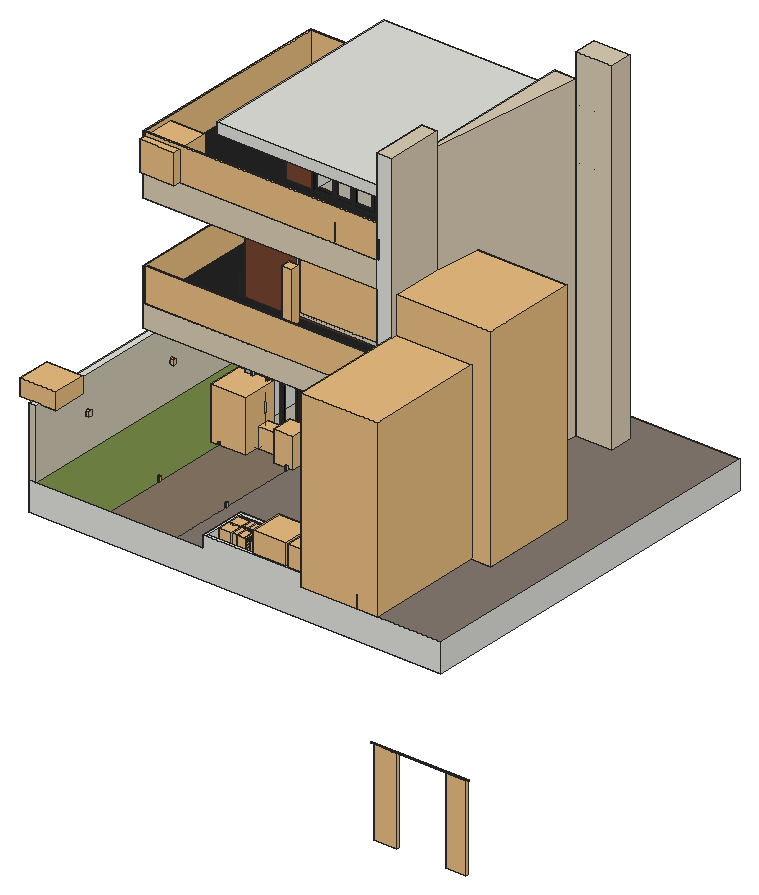
# SketchUp Ruby script. Lengths in inches.
U = 1.inch
M = Sketchup.active_model
def pt(a) = Geom::Point3d.new(a.map { |v| v * U })
def face(e, loops, mat)
  f = e.add_face(loops[0].map { |a| pt(a) })
  loops[1..].each { |l| e.add_face(l.map { |a| pt(a) }).erase! }
  f.material = f.back_material = mat if mat
  f
end
# faces: each face lists its corners as indices into pts; further lists are holes
def faces(e, pts, list, mat = nil) = list.each { |f| face(e, (f[0].is_a?(Array) ? f : [f]).map { |l| l.map { |i| pts[i] } }, mat) }
# xy, xz, yz: faces in a plane at the given z, y or x. An outline is a flat list of corners, or four numbers for a rectangle; further outlines are holes
def ring(l) = l.size == 4 ? [[l[0], l[1]], [l[2], l[1]], [l[2], l[3]], [l[0], l[3]]] : l.each_slice(2).to_a
def flat(e, list, mat, &to3) = list.each { |f| face(e, (f[0].is_a?(Array) ? f : [f]).map { |l| ring(l).map { |u, v| to3.(u, v) } }, mat) }
def xy(e, z, list, mat = nil) = flat(e, list, mat) { |x, y| [x, y, z] }
def xz(e, y, list, mat = nil) = flat(e, list, mat) { |x, z| [x, y, z] }
def yz(e, x, list, mat = nil) = flat(e, list, mat) { |y, z| [x, y, z] }
def lines(e, pts, list) = list.each { |a, b| e.add_line(pt(pts[a]), pt(pts[b])) }
# prism: a flat outline (further loops are holes) pulled along v
def prism(e, loops, v, mat = nil)
  f = face(e, loops, mat); d = Geom::Vector3d.new(v.map { |x| x * U })
  f.pushpull(f.normal.samedirection?(d) ? d.length : -d.length)
end
def box(e, o, s, mat = nil) = prism(e, [[o, [o[0] + s[0], o[1], o[2]], [o[0] + s[0], o[1] + s[1], o[2]], [o[0], o[1] + s[1], o[2]]]], [0, 0, s[2]], mat)
def at(x, y, z, deg = 0) = Geom::Transformation.translation(pt([x, y, z])) * Geom::Transformation.rotation(ORIGIN, Z_AXIS, deg.degrees)
def axes(o, x, y, z) = Geom::Transformation.new([*x, 0, *y, 0, *z, 0, *pt(o).to_a, 1])
def part(name) = M.definitions.add(name)
# library, detail: a bought-in or finely detailed component or shape, given as its bounding box
def library(name, o, s) = part(name).tap { |d| box(d.entities, o, s) }
def detail(e, o, s) = box(e.add_group.entities, o, s)
def put(e, d, t, mat = nil) = e.add_instance(d, t).tap { |i| i.material = mat if mat }
def group(e, t, mat = nil) = e.add_group.tap { |g| g.transformation = t; g.material = mat if mat }.entities
root = M.entities
M.materials.add("AWS- Aluminium").color = [33, 33, 33]
M.materials.add("Door-black").color = [0, 0, 0]
M.materials.add("Generic").color = [184, 178, 163]
M.materials.add("Grass C 200cm").color = [117, 136, 71]
M.materials.add("Gravel D01 80cm").color = [133, 121, 111]
M.materials.add("Stone B 150cm").color = [135, 119, 102]
M.materials.add("Stone Beige 01 200cm\#2").color = [209, 202, 180]
M.materials.add("Stucco E01 50cm").color = [117, 69, 47]
M.materials.add("WallPaint_FineGrain_01_White_1m").color = [186, 186, 184]
M.materials.add("[0136_Charcoal]").color = [35, 35, 35]
M.materials.add("beige").color = [218, 205, 180]
M.materials.add("clear_glass").color = [0, 0, 0]
M.materials["clear_glass"].alpha = 0
M.materials.add("very light warm off").color = [203, 196, 183]
c1 = library("Door 243 066",[-40.92,-2.1,0],[81.84,4.2,82.99])
c2 = library("Back Drop",[0,0,0],[82.68,2.27,107.48])
c3 = part("Tlon Cubo 590 Ceiling 152 004")
xy(c3.entities,-3.04,[[-11.22,-11.22,-11.22,11.22,11.22,-11.22],[11.22,-11.22,-11.22,11.22,11.22,11.22]])
xy(c3.entities,0,[[-11.61,-11.61,11.61,-11.61,-11.61,11.61],[11.61,-11.61,11.61,11.61,-11.61,11.61]])
xz(c3.entities,-11.61,[[-11.61,-3.79,11.61,-3.79,-11.61,0],[11.61,-3.79,11.61,0,-11.61,0]])
xz(c3.entities,-10.98,[[-10.98,-3.66,-10.98,-3.24,10.98,-3.24],[-10.98,-3.66,10.98,-3.24,10.98,-3.66]])
xz(c3.entities,10.98,[[-10.98,-3.66,10.98,-3.24,-10.98,-3.24],[-10.98,-3.66,10.98,-3.66,10.98,-3.24]])
xz(c3.entities,11.61,[[-11.61,-3.79,-11.61,0,11.61,0],[-11.61,-3.79,11.61,0,11.61,-3.79]])
yz(c3.entities,-11.61,[[-11.61,-3.79,-11.61,0,11.61,0],[-11.61,-3.79,11.61,0,11.61,-3.79]])
yz(c3.entities,-10.98,[[-10.98,-3.66,10.98,-3.66,-10.98,-3.24],[10.98,-3.66,10.98,-3.24,-10.98,-3.24]])
yz(c3.entities,10.98,[[-10.98,-3.66,-10.98,-3.24,10.98,-3.66],[10.98,-3.66,-10.98,-3.24,10.98,-3.24]])
yz(c3.entities,11.61,[[-11.61,-3.79,11.61,-3.79,-11.61,0],[11.61,-3.79,11.61,0,-11.61,0]])
p = [[-11.61,-11.61,-3.79],[-11.61,11.61,-3.79],[-10.98,10.98,-3.66],[-10.98,-10.98,-3.66],[11.61,-11.61,-3.79],[10.98,-10.98,-3.66],
  [11.61,11.61,-3.79],[10.98,10.98,-3.66]]
faces(c3.entities,p,[[0,1,2],[2,3,0],[4,0,3],[3,5,4],[6,4,5],[5,7,6],[2,1,6],[6,7,2]])
c4 = library("Lugstar Premium LED 152 063",[-3.77,-3.75,-3.3125],[7.54,7.53,3.3125])
c5 = library("Lamp Ceiling 35-55",[-2.36,-2.36,-1.36],[4.72,4.72,1.36])
c6 = library("Rossi Sofa",[-52.17,-19.09,0],[104.34,38.18,34.45])
c7 = library("Bed 49-33",[-39.37,-46.12,0],[78.74,92.24,55.51])
c8 = library("Wardrobe 27-03",[-60.67,-12.8,0],[121.34,25.6,93.86])
c9 = library("Grad Meeting",[-51.09,-20.37,0],[102.18,40.74,30.85])
c10 = library("Potted plant",[0,0,0],[10.9,9.89,25.73])
c11 = library("Curtain rod",[-106.15,-0.12,-0.12],[207.64,1.02,1.02])
c12 = library("Curtain panel",[52.48,-0.06,0],[27.24,5.33,103.27])
c13 = part("Curtains and rod")
put(c13.entities,c11,at(101.49,3.47,111.75,-180))
put(c13.entities,c12,axes([150,6.58,3.41],[-1.81149,0,0],[0,-1,0],[0,0,1.04934]))
put(c13.entities,c12,axes([74.4,6.77,3.41],[1.6095,0,0],[0,-1,0],[0,0,1.04934]))
c14 = library("BED+7",[-211.22,-92.85,196.6875],[87.15,98.53,46.62])
c15 = library("wardrobe+",[-8.26,0,0],[41.85,97.64,98.43])
c16 = library("Glass+Railings(black+Handrails)",[-57.04,-132.55,0],[169.29,2.52,28.17])
c17 = library("Tall Climbing Plant 50-13",[-4.09,-3.9375,0],[8.41,8.24,37.49])
c18 = library("Interior Plant 273 009 002",[-22.5,-22.44,0],[44.9,45.03,65.72])
c19 = library("Potted Plant 15",[-14.27,-11.47,0],[24.64,26.73,38.28])
c20 = library("Indoor Plant 009",[-22.3,-24.54,0],[44.36,48.53,38])
c21 = library("Wall Panel 104-19",[-41.37,-3.09,0],[82.74,3.09,105.27])
c22 = library("Sedum Plant 66-24",[-7.97,-7.95,0.04],[16.42,16.31,19.57])
c23 = library("Large Boxwood Plant 66-28",[-21.37,-20.87,0.32],[41.28,41.36,41.23])
c24 = library("Planted timber trough",[0,0,0],[56.02,15.3,25.28])
c25 = library("3d tree - Pine",[-19.9,-19.35,0],[38.46,38.42,75.98])
c26 = library("3d tree - apple tree",[-40.02,-45.64,0],[79.61,84.93,119.53])
c27 = library("Lamp Wall Outdoor 94-02",[-1.89,-4.65,-3.17],[3.78,4.65,6.35])
c28 = library("Hakonechloa Macra Green Forest Grass 003",[-38.79,-36.76,-0.98],[79.26,72.43,36.83])
c29 = library("Dome Light",[-12,-12,0],[24,24,12])
c30 = library("Lamp Ceiling 114-44",[-1.26,-1.26,-3.9375],[2.52,2.52,3.9375])
c31 = part("Group179\#1")
p = [[0,0,0],[0,0,-12.9],[-1.75,0,-12.9],[11.37,-30.39,0],[-11.37,-30.39,0],[11.37,30.39,0],
  [11.37,0,0],[-11.37,30.39,0],[1.75,0,-12.9],[-11.37,0,0],[0,0,-20.88]]
lines(c31.entities,p,[[0,1],[1,2],[3,4],[5,6],[7,5],[1,8],[9,0],[0,6],[8,10],[4,9],[6,3],[2,10],
  [9,7]])
c32 = part("Rectangle Light")
put(c32.entities,c31,at(0,0,0))
c33 = library("Group\#2",[-0.5,-0.5,-0.1],[95.1,119.5,0.2])
c34 = library("Group\#3",[-0.5,-0.5,-0.1],[120.5,81.4,0.2])
c35 = library("Mesh Light\#3",[-0.5,-0.5,-0.1],[1,1,0.2])
c36 = library("Group\#6",[0,0,0],[125.67,2.7,109.8])
c37 = part("Door glazing pane")
box(c37.entities,[0,-0.39,0],[29.625,0.39,87.4],"clear_glass")
c38 = part("Door infill panel")
prism(c38.entities,[[[30.41,1.18,88.1875],[30.41,1.18,0],[0,1.18,0],[0,1.18,88.1875]],[[30.02,1.18,0.39],[30.02,1.18,87.8],[0.39,1.18,87.8],[0.39,1.18,0.39]]],[0,-1.18,0],"Door-black")
put(c38.entities,c37,at(0.39,0.79,0.39))
c39 = part("Framed door panel")
prism(c39.entities,[[[36.71,1.57,0],[0,1.57,0],[0,1.57,94.49],[36.71,1.57,94.49]],[[33.5625,1.57,3.15],[33.5625,1.57,91.34],[3.15,1.57,91.34],[3.15,1.57,3.15]]],[0,-1.57,0],"AWS- Aluminium")
put(c39.entities,c38,at(3.15,0.2,3.15),"AWS- Aluminium")
c40 = part("Recessed door pull")
xy(c40.entities,0,[[0,0,1.18,0.39]])
xy(c40.entities,0.1875,[[0.1875,0.2,0.99,0.39]])
xy(c40.entities,5.36,[[0.1875,0.2,0.99,0.59]])
xy(c40.entities,7.68,[[0.1875,0.39,0.99,0.59]])
xy(c40.entities,7.875,[[0,0,1.18,0.39]])
xz(c40.entities,0,[[0,0,1.18,7.875]])
xz(c40.entities,0.2,[[0.1875,0.1875,0.99,5.36]])
xz(c40.entities,0.39,[[[0,0,1.18,7.875],[0.1875,0.1875,0.99,7.68]]])
xz(c40.entities,0.59,[[0.1875,5.36,0.99,7.68]])
yz(c40.entities,0,[[0,0,0.39,7.875]])
yz(c40.entities,0.1875,[[0.2,0.1875,0.39,5.36],[0.39,5.36,0.59,7.68]])
yz(c40.entities,0.99,[[0.2,0.1875,0.39,5.36],[0.39,5.36,0.59,7.68]])
yz(c40.entities,1.18,[[0,0,0.39,7.875]])
c41 = part("Group\#16")
prism(c41.entities,[[[144.49,3.9375,98.43],[144.49,3.9375,0],[0,3.9375,0],[0,3.9375,98.43]],[[1.97,3.9375,1.97],[142.52,3.9375,1.97],[142.52,3.9375,96.46],[1.97,3.9375,96.46]]],[0,-3.9375,0],"AWS- Aluminium")
put(c41.entities,c39,at(105.81,0,1.97))
put(c41.entities,c39,at(72.34,1.77,1.97))
put(c41.entities,c39,axes([38.68,0,1.97],[-1,0,0],[0,1,0],[0,0,1]))
put(c41.entities,c39,axes([72.15,1.77,1.97],[-1,0,0],[0,1,0],[0,0,1]))
put(c41.entities,c40,at(69.98,3.35,41.96))
put(c41.entities,c40,at(73.33,3.35,41.96))
c42 = library("Mesh Light\#2",[-0.5,-0.5,-0.1],[1,1,0.2])
xy(root,27.61,[[0,0,0,409.9,102.7,409.9,102.7,475.9,525.7,475.9,525.7,0]])
xy(root,64.21,[[188.05,211.64,264.4,211.64,264.4,215.4,342.7,215.4,342.7,409.9,102.7,409.9,102.7,215.4,188.05,215.4],[342.7,215.4,348.3,215.4,369.5,409.9,342.7,409.9],[102.7,409.9,369.5,475.9],[369.5,409.9,415.4,438.9]])
xy(root,64.21,[[9,0,102.7,388.4],[225.6875,3.72,414.64,55.78]],"Grass C 200cm")
xy(root,64.21,[[188.05,0,221.97,0,221.97,59.5,418.37,59.5,418.37,0,525.7,0,525.7,475.9,369.5,475.9,369.5,438.9,415.4,438.9,415.4,409.9,369.5,409.9,348.3,215.4,264.4,215.4,264.4,211.64,188.05,211.64]],"Gravel D01 80cm")
xy(root,64.21,[[102.7,0,188.05,215.4]],"Stone B 150cm")
xy(root,67.7,[[188.05,211.64,264.4,211.64,264.4,353.9,113.69,353.9,113.69,215.4,188.05,215.4]],"Generic")
xy(root,79.81,[[[221.97,0,418.37,59.5],[225.6875,3.72,414.64,55.78]]])
xy(root,152.31,[[0,0,9,0,9,388.4,102.7,388.4,102.7,409.9,0,409.9]])
xy(root,183.71,[[[113.69,215.4,264.4,353.9],[125.79,244.05,245.29,324.45]],[127.17,245.4375,243.91,323.07]],"very light warm off")
xy(root,185.71,[[[30.7,143.4,30.7,409.9,102.7,409.9,102.7,215.4,348.3,215.4,348.3,143.4],[42.07,151.03,338.07,151.03,338.07,197.73,89.77,197.73,89.77,388.63,42.07,388.63]],[44,152.97,44,386.7,87.84,386.7,87.84,195.8,336.14,195.8,336.14,152.97]],"beige")
xy(root,215.21,[[30.7,143.4,328.78,143.4,328.78,215.4,102.7,215.4,102.7,409.9,30.7,409.9]],"[0136_Charcoal]")
xy(root,221.71,[[172.99,215.4,297.55,369.6]],"Generic")
xy(root,331.5,[[[172.99,215.4,297.55,369.6],[193.83,232.75,287.93,351.25]],[195.38,234.3,286.38,349.7]],"very light warm off")
xy(root,335.21,[[[30.7,143.4,30.7,409.9,102.7,409.9,102.7,215.4,328.78,215.4,328.78,143.4],[47.43,152.79,318.43,152.79,318.43,197.29,94.03,197.29,94.03,394.99,47.43,394.99]],[49.49,154.85,49.49,392.94,91.98,392.94,91.98,195.24,316.38,195.24,316.38,154.85]],"beige")
xy(root,368.91,[[30.7,143.4,328.78,143.4,328.78,215.4,155.8,215.4,155.8,409.9,30.7,409.9]],"[0136_Charcoal]")
xy(root,372.625,[[196.52,215.4,291.78,282.9]],"Generic")
xy(root,437.1875,[[196.52,215.4,291.78,282.9]],"very light warm off")
xy(root,440.91,[[155.8,215.4,342.7,409.9]])
xy(root,440.91,[[125.3,143.4,125.3,409.9,155.8,409.9,155.8,215.4,328.78,215.4,328.78,143.4]],"beige")
xy(root,454.41,[[125.3,143.4,328.78,143.4,328.78,215.4,342.7,215.4,342.7,409.9,125.3,409.9]])
xy(root,473.21,[[342.7,215.4,348.3,215.4,369.5,409.9,342.7,409.9]],"beige")
xy(root,491.13,[[328.78,143.4,348.3,215.4]],"beige")
xy(root,504.01,[[369.5,409.9,415.4,438.9]],"beige")
xz(root,0,[[0,27.61,525.7,27.61,525.7,64.21,418.37,64.21,418.37,79.81,221.97,79.81,221.97,64.21,0,64.21]])
xz(root,0,[[0,64.21,9,152.31]],"Stone Beige 01 200cm\#2")
xz(root,3.72,[[225.6875,64.21,414.64,79.81]])
xz(root,55.78,[[225.6875,64.21,414.64,79.81]])
xz(root,59.5,[[221.97,64.21,418.37,79.81]])
xz(root,143.4,[[328.78,185.71,348.3,491.13],[125.3,440.91,328.78,454.41]])
xz(root,143.4,[[30.7,185.71,328.78,215.21],[30.7,335.21,328.78,368.91]],"beige")
xz(root,211.64,[[188.05,64.21,264.4,67.7]])
xz(root,215.4,[[342.7,64.21,348.3,185.71],[188.05,183.71,264.4,185.71],[342.7,185.71,348.3,215.21],[342.7,215.21,348.3,335.21],[342.7,335.21,348.3,368.91],
  [[192.8,368.91,295.5,440.91],[196.52,372.625,291.78,437.1875]],[342.7,368.91,348.3,473.21],[328.78,440.91,342.7,454.41],[328.78,454.41,328.78,491.13,348.3,491.13,348.3,473.21,342.7,473.21,342.7,454.41]])
xz(root,215.4,[[111.7,64.21,188.05,64.21,188.05,67.7,113.69,67.7,113.69,183.71,188.05,183.71,188.05,185.71,111.7,185.71]],"Generic")
xz(root,215.4,[[102.7,215.21,328.78,215.21,328.78,335.21,301.25,335.21,301.25,218.01,169.29,218.01,169.29,335.21,102.7,335.21],[155.8,368.91,192.8,440.91],[295.5,368.91,328.78,440.91]],"Stucco E01 50cm")
xz(root,215.4,[[102.7,64.21,111.7,185.71]],"WallPaint_FineGrain_01_White_1m")
xz(root,215.4,[[264.4,64.21,342.7,185.71],[[169.29,218.01,301.25,335.21],[172.99,221.71,297.55,331.5]]],"beige")
xz(root,282.9,[[196.52,372.625,291.78,437.1875]])
xz(root,353.9,[[113.69,67.7,264.4,183.71]])
xz(root,369.6,[[172.99,221.71,297.55,331.5]])
xz(root,388.4,[[9,64.21,102.7,152.31]],"Stone Beige 01 200cm\#2")
xz(root,409.9,[[0,27.61,102.7,152.31],[102.7,64.21,102.7,185.71,30.7,185.71,30.7,215.21,102.7,215.21,102.7,335.21,30.7,335.21,30.7,368.91,155.8,368.91,155.8,440.91,342.7,440.91,342.7,473.21,369.5,473.21,369.5,64.21],[125.3,440.91,342.7,454.41]])
xz(root,409.9,[[369.5,64.21,415.4,504.01]],"beige")
xz(root,417,[[373.67,378.06,393.43,443.61]])
xz(root,438.9,[[369.5,64.21,415.4,504.01]])
xz(root,475.9,[[102.7,27.61,525.7,64.21]])
yz(root,0,[[0,27.61,409.9,152.31]],"Stone Beige 01 200cm\#2")
yz(root,9,[[0,64.21,388.4,152.31]],"Stone Beige 01 200cm\#2")
yz(root,30.7,[[143.4,185.71,409.9,215.21],[143.4,335.21,409.9,368.91]],"beige")
yz(root,102.7,[[409.9,27.61,475.9,64.21],[388.4,64.21,409.9,152.31]])
yz(root,102.7,[[215.4,64.21,215.4,185.71,409.9,185.71,409.9,152.31,388.4,152.31,388.4,64.21],[215.4,215.21,409.9,335.21]],"beige")
yz(root,113.69,[[215.4,67.7,353.9,183.71]])
yz(root,125.3,[[143.4,440.91,409.9,454.41]])
yz(root,155.8,[[215.4,368.91,409.9,440.91]])
yz(root,172.99,[[215.4,221.71,369.6,331.5]])
yz(root,188.05,[[211.64,64.21,215.4,67.7]])
yz(root,196.52,[[215.4,372.625,282.9,437.1875]])
yz(root,221.97,[[0,64.21,59.5,79.81]])
yz(root,225.6875,[[3.72,64.21,55.78,79.81]])
yz(root,264.4,[[211.64,64.21,215.4,67.7],[215.4,67.7,353.9,183.71]])
yz(root,291.78,[[215.4,372.625,282.9,437.1875]])
yz(root,297.55,[[215.4,221.71,369.6,331.5]])
yz(root,328.78,[[143.4,440.91,215.4,454.41],[143.4,454.41,215.4,491.13]])
yz(root,328.78,[[143.4,215.21,215.4,335.21],[143.4,368.91,215.4,440.91]],"Stucco E01 50cm")
yz(root,342.7,[[215.4,440.91,409.9,454.41],[215.4,454.41,409.9,473.21]])
yz(root,348.3,[[143.4,185.71,215.4,491.13]],"beige")
yz(root,369.5,[[409.9,64.21,438.9,504.01]])
yz(root,414.64,[[3.72,64.21,55.78,79.81]])
yz(root,415.4,[[409.9,64.21,438.9,504.01]],"beige")
yz(root,418.37,[[0,64.21,59.5,79.81]])
yz(root,525.7,[[0,27.61,475.9,64.21]])
p = [[369.5,409.9,473.21],[348.3,215.4,473.21],[348.3,215.4,368.91],[348.3,215.4,335.21],[348.3,215.4,215.21],[348.3,215.4,185.71],
  [348.3,215.4,64.21],[369.5,409.9,64.21],[342.7,215.4,215.21],[328.78,215.4,215.21],[342.7,215.4,335.21],[328.78,215.4,335.21],
  [315.58,215.4,215.21],[315.58,215.4,185.71],[315.58,215.4,368.91],[315.58,215.4,335.21],[342.7,215.4,368.91],[328.78,215.4,368.91],
  [393.43,409.9,378.06],[393.43,417,378.06],[373.67,409.9,378.06],[373.67,417,378.06],[393.43,409.9,443.61],[393.43,417,443.61],
  [373.67,409.9,443.61],[373.67,417,443.61]]
faces(root,p,[[0,1,2,3,4,5,6,7]],"beige")
lines(root,p,[[8,9],[10,11],[12,13],[14,15],[16,17],[18,19],[20,21],[22,23],[24,25]])
put(root,c1,axes([226.2,213.74,67.85],[0.93372,0,0],[0,1,0],[0,0,1.42006]))
put(root,c2,axes([264.41,213.11,64.21],[1.007,0,0],[0,1,0],[0,0,1.12955]))
put(root,c3,at(214.16,265.65,183.71))
put(root,c3,at(153.26,268.94,183.71))
put(root,c4,axes([240.06,299.51,330.79],[0.84,0,0],[0,0.84,0],[0,0,0.5964]))
put(root,c4,axes([240.06,291.95,330.79],[0.84,0,0],[0,0.84,0],[0,0,0.5964]))
put(root,c4,axes([240.06,284.39,330.79],[0.84,0,0],[0,0.84,0],[0,0,0.5964]))
put(root,c4,axes([240.06,276.83,330.79],[0.84,0,0],[0,0.84,0],[0,0,0.5964]))
put(root,c4,axes([240.06,254.41,437.1875],[0.84,0,0],[0,0.84,0],[0,0,0.42]))
put(root,c4,axes([240.06,246.85,437.1875],[0.84,0,0],[0,0.84,0],[0,0,0.42]))
put(root,c4,axes([278.26,231.73,437.1875],[0.84,0,0],[0,0.84,0],[0,0,0.42]))
put(root,c4,axes([240.06,239.29,437.1875],[0.84,0,0],[0,0.84,0],[0,0,0.42]))
put(root,c5,at(264.97,249.28,331.5))
put(root,c5,at(213.37,249.28,331.5))
put(root,c5,at(213.37,321.28,331.5))
put(root,c5,at(271.17,321.28,331.5))
put(root,c4,axes([210.66,231.73,437.1875],[0.84,0,0],[0,0.84,0],[0,0,0.42]))
put(root,c4,axes([210.66,266.83,437.1875],[0.84,0,0],[0,0.84,0],[0,0,0.42]))
put(root,c4,axes([280.96,266.83,437.1875],[0.84,0,0],[0,0.84,0],[0,0,0.42]))
put(root,c6,at(174.65,303.66,67.7))
put(root,c7,axes([267.07,304.1875,221.1875],[0,-0.6608,0],[0.6608,0,0],[0,0,0.6608]))
put(root,c8,axes([250.98,332.98,230.54],[0.68,0,0],[0,0.68,0],[0,0,0.68]))
put(root,c9,axes([193.11,334.24,230.54],[0.32521,0,0],[0,0.3654,0],[0,0,0.60291]))
put(root,c10,at(286.28,255.97,221.71))
put(root,c13,axes([896.21,-575.64,218.28],[0.59986,0,0],[0,0.4895,0],[0,0,1.00509]))
put(root,c14,axes([205.82,228.03,292.57],[-0.407,0,0],[0,-0.407,0],[0,0,0.407]))
put(root,c15,axes([197.89,282.91,372.625],[0,-0.7224,0],[0.6708,0,0],[0,0,0.57142]))
put(root,c16,axes([132.41,275.95,215.19],[1.74947,0,0],[0,1,0],[0,0,1.5]))
put(root,c16,axes([-99.34,231.38,215.2],[0,1.54231,0],[-1,0,0],[0,0,1.5]))
put(root,c16,axes([132.42,275.95,368.9],[1.74947,0,0],[0,1,0],[0,0,1.5]))
put(root,c16,axes([-99.33,232.26,368.91],[0,1.55773,0],[-1,0,0],[0,0,1.5]))
put(root,c16,axes([73.56,539.9375,368.9],[0.73268,0,0],[0,1,0],[0,0,1.5]))
put(root,c17,axes([170.31,203.11,215.21],[1.5,0,0],[0,1.43,0],[0,0,1.74]))
put(root,c17,axes([308.41,203.11,215.21],[1.5,0,0],[0,1.43,0],[0,0,1.74]))
put(root,c18,at(114.8,197.04,64.21))
put(root,c19,at(181.98,191.78,64.21))
put(root,c19,at(252.04,192.5625,64.21))
put(root,c20,at(81.18,387.03,215.21))
put(root,c20,at(55.47,159.23,368.91))
put(root,c21,axes([73.11,404.5,216.08],[0.96552,0,0],[0,1,0],[0,0,1.13166]))
put(root,c21,axes([70.95,392.17,335.21],[0.49825,0,0],[0,0,0.16183],[0,-2.25471,0]))
put(root,c21,axes([313.74,174.22,335.45],[0,-0.46889,0],[0,0,0.24254],[-2.11065,0,0]))
put(root,c21,axes([65.29,390.29,186.11],[0.51355,0,0],[0,0,0.28159],[0,-2.23216,0]))
put(root,c21,axes([336.14,173.16,186.11],[0,-0.47845,0],[0,0,0.24254],[-2.37113,0,0]))
put(root,c22,at(253.9375,38.61,64.21))
put(root,c22,at(261.61,37.07,64.41))
put(root,c22,at(273.76,37.07,64.41))
put(root,c22,at(253.9375,23.53,64.21))
put(root,c22,at(273.76,21.99,64.41))
put(root,c22,at(261.61,21.99,64.41))
put(root,c23,at(305.54,23.34,64.21))
put(root,c23,at(349.87,23,64.21))
put(root,c23,at(393.73,27.96,64.21))
put(root,c22,at(238.3125,21.99,64.41))
put(root,c22,at(238.3125,37.07,64.41))
put(root,c24,at(125.83,193.09,64.21))
put(root,c24,at(35.32,144.9375,218.48))
put(root,c24,at(85.42,144.9375,218.48))
put(root,c24,at(135.62,144.9375,218.48))
put(root,c24,at(174.74,144.45,369.3))
put(root,c24,at(224.84,144.45,369.3))
put(root,c24,at(275.04,144.45,369.3))
put(root,c25,axes([405.16,210.44,64.21],[-3.18383,0,0],[0,-3.16,0],[0,0,3.5346]))
put(root,c26,axes([396.23,100.02,64.21],[1.2221,0,0],[0,2.1917,0],[0,0,1.8584]))
put(root,c27,at(57.14,388.4,110.59))
put(root,c27,at(9,80.41,109.47,90))
put(root,c27,at(9,215.01,109.47,90))
put(root,c28,axes([6.01,27.86,151.9],[0.58,0,0],[0,0.58,0],[0,0,0.58]))
put(root,c28,at(0,393.39,152.31))
put(root,c29,at(345.9,137.51,75.8))
put(root,c30,axes([307.62,166.55,185.81],[1,0,0],[0,1,0],[0,0,1.27]))
put(root,c30,axes([65.92,166.55,185.81],[1,0,0],[0,1,0],[0,0,1.27]))
put(root,c30,axes([65.92,370.05,185.81],[1,0,0],[0,1,0],[0,0,1.27]))
put(root,c30,axes([304.42,166.55,185.81],[1,0,0],[0,1,0],[0,0,1.27]))
put(root,c30,axes([68.02,166.75,185.81],[1,0,0],[0,1,0],[0,0,1.27]))
put(root,c30,axes([62.92,370.05,185.81],[1,0,0],[0,1,0],[0,0,1.27]))
put(root,c30,axes([155.52,166.55,185.81],[1,0,0],[0,1,0],[0,0,1.27]))
put(root,c30,axes([216.32,166.55,185.81],[1,0,0],[0,1,0],[0,0,1.27]))
put(root,c30,axes([300.42,166.51,335.31],[1,0,0],[0,1,0],[0,0,1.27]))
put(root,c30,axes([297.22,166.51,335.31],[1,0,0],[0,1,0],[0,0,1.27]))
put(root,c30,axes([155.52,166.55,335.31],[1,0,0],[0,1,0],[0,0,1.27]))
put(root,c30,axes([216.32,166.55,335.31],[1,0,0],[0,1,0],[0,0,1.27]))
put(root,c30,axes([65.92,370.05,335.31],[1,0,0],[0,1,0],[0,0,1.27]))
put(root,c30,axes([65.92,169.45,335.31],[1,0,0],[0,1,0],[0,0,1.27]))
put(root,c30,axes([62.92,370.05,335.31],[1,0,0],[0,1,0],[0,0,1.27]))
put(root,c30,axes([65.92,166.55,335.31],[1,0,0],[0,1,0],[0,0,1.27]))
put(root,c30,axes([137.47,171.53,440.91],[1,0,0],[0,1,0],[0,0,1.27]))
put(root,c30,axes([137.47,168.63,440.91],[1,0,0],[0,1,0],[0,0,1.27]))
put(root,c30,axes([299.87,171.53,440.91],[1,0,0],[0,1,0],[0,0,1.27]))
put(root,c30,axes([299.87,168.63,440.91],[1,0,0],[0,1,0],[0,0,1.27]))
put(root,c30,axes([226.77,168.63,440.91],[1,0,0],[0,1,0],[0,0,1.27]))
put(root,c30,axes([226.77,171.53,440.91],[1,0,0],[0,1,0],[0,0,1.27]))
put(root,c30,axes([137.47,263.93,440.91],[1,0,0],[0,1,0],[0,0,1.27]))
put(root,c30,axes([137.47,261.03,440.91],[1,0,0],[0,1,0],[0,0,1.27]))
put(root,c30,axes([137.47,378.73,440.91],[1,0,0],[0,1,0],[0,0,1.27]))
put(root,c30,axes([137.47,375.83,440.91],[1,0,0],[0,1,0],[0,0,1.27]))
put(root,c30,axes([65.92,282.05,335.31],[1,0,0],[0,1,0],[0,0,1.27]))
put(root,c30,axes([158.12,166.55,185.81],[1,0,0],[0,1,0],[0,0,1.27]))
put(root,c30,axes([219.29,166.55,185.81],[1,0,0],[0,1,0],[0,0,1.27]))
put(root,c30,axes([101.87,176.5,69.06],[1,0,0],[0,1,0],[0,0,1.27]))
put(root,c30,axes([63.29,281.15,335.13],[1,0,0],[0,1,0],[0,0,1.27]))
put(root,c30,axes([157.92,166.55,335.31],[1,0,0],[0,1,0],[0,0,1.27]))
put(root,c30,axes([219.42,166.55,335.31],[1,0,0],[0,1,0],[0,0,1.27]))
put(root,c30,axes([67.7,169.45,335.31],[1,0,0],[0,1,0],[0,0,1.27]))
put(root,c30,axes([67.7,166.55,335.31],[1,0,0],[0,1,0],[0,0,1.27]))
put(root,c30,axes([139.79,170.64,440.76],[1,0,0],[0,1,0],[0,0,1.27]))
put(root,c30,axes([187.03,80.6,69.06],[1,0,0],[0,1,0],[0,0,1.27]))
put(root,c30,axes([101.87,80.6,69.06],[1,0,0],[0,1,0],[0,0,1.27]))
put(root,c30,axes([187.03,176.5,69.06],[1,0,0],[0,1,0],[0,0,1.27]))
put(root,c32,axes([84.3,291.68,215.22],[1,0,0],[0,-1,0],[0,0,-1.89]))
put(root,c32,axes([134.38,168.16,215.21],[0,-1,0],[-1,0,0],[0,0,-2.835]))
put(root,c32,axes([142.43,198.74,67.83],[0,-1,0],[-1,0,0],[0,0,-2.835]))
g1 = group(root,at(30.7,409.9,215.21),"WallPaint_FineGrain_01_White_1m")
box(g1,[0,-5.4,0],[72,5.4,120])
put(root,c33,at(193.83,232.75,331.5))
put(root,c34,at(125.79,244.05,183.71))
g2 = group(root,at(42.07,151.03,185.71))
xy(g2,0,[[[0,0,0,237.6,47.7,237.6,47.7,46.7,296,46.7,296,0],[1.93,1.93,294.07,1.93,294.07,44.77,45.77,44.77,45.77,235.67,1.93,235.67]]],"beige")
put(g2,c35,axes([148,118.8,0],[297,0,0],[0,238.6,0],[0,0,1]))
put(root,c36,at(171.875,215.4,221.71))
put(root,c41,axes([111.51,220.42,67.7],[0.53539,0,0],[0,-1.56765,0],[0,0,1.17869]))
put(root,c41,axes([192.51,217.12,368.91],[0.71208,0,0],[0,-1.56765,0],[0,0,0.73152]))
g3 = group(root,at(47.43,152.79,335.21))
xy(g3,0,[[[0,0,0,242.2,46.6,242.2,46.6,44.5,271,44.5,271,0],[2.05,2.05,268.95,2.05,268.95,42.45,44.55,42.45,44.55,240.15,2.05,240.15]]],"beige")
put(g3,c42,axes([135.5,121.1,0],[272,0,0],[0,243.2,0],[0,0,1]))
